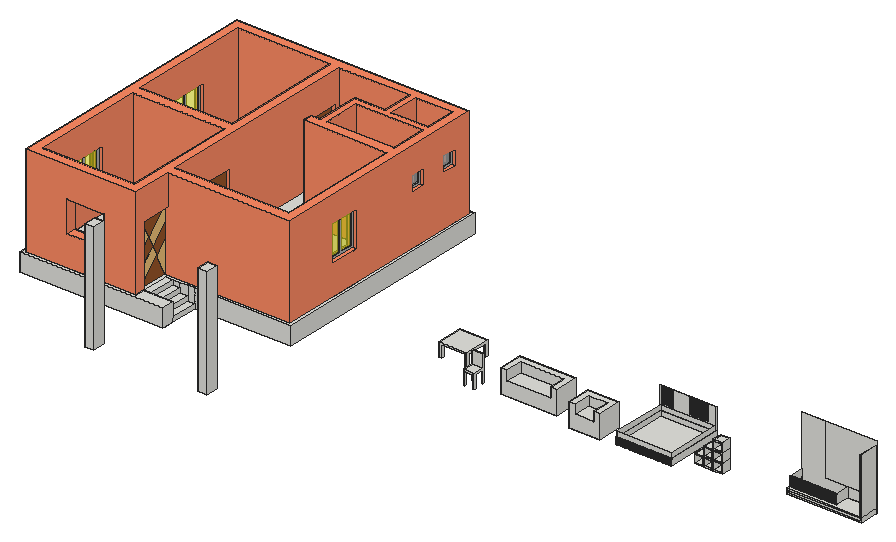
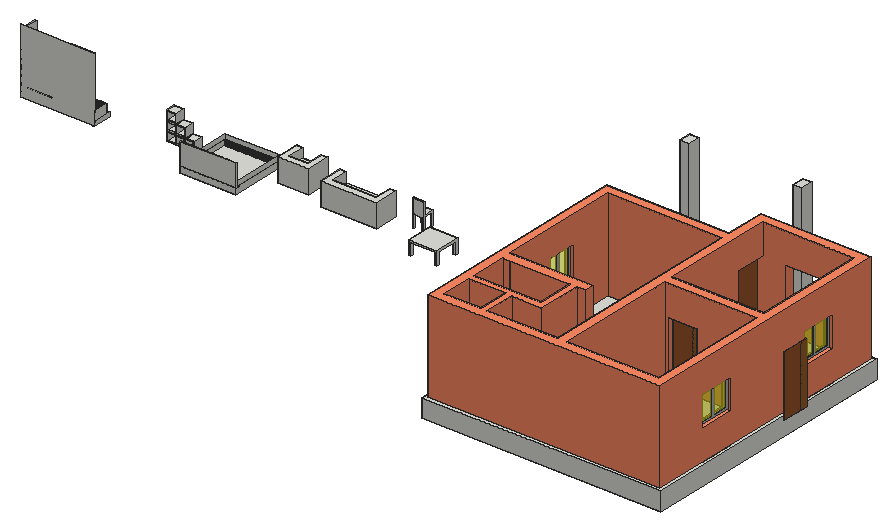
# SketchUp Ruby script. Lengths in inches.
U = 1.inch
M = Sketchup.active_model
def pt(a) = Geom::Point3d.new(a.map { |v| v * U })
def face(e, loops, mat)
  f = e.add_face(loops[0].map { |a| pt(a) })
  loops[1..].each { |l| e.add_face(l.map { |a| pt(a) }).erase! }
  f.material = f.back_material = mat if mat
  f
end
# faces: each face lists its corners as indices into pts; further lists are holes
def faces(e, pts, list, mat = nil) = list.each { |f| face(e, (f[0].is_a?(Array) ? f : [f]).map { |l| l.map { |i| pts[i] } }, mat) }
# xy, xz, yz: faces in a plane at the given z, y or x. An outline is a flat list of corners, or four numbers for a rectangle; further outlines are holes
def ring(l) = l.size == 4 ? [[l[0], l[1]], [l[2], l[1]], [l[2], l[3]], [l[0], l[3]]] : l.each_slice(2).to_a
def flat(e, list, mat, &to3) = list.each { |f| face(e, (f[0].is_a?(Array) ? f : [f]).map { |l| ring(l).map { |u, v| to3.(u, v) } }, mat) }
def xy(e, z, list, mat = nil) = flat(e, list, mat) { |x, y| [x, y, z] }
def xz(e, y, list, mat = nil) = flat(e, list, mat) { |x, z| [x, y, z] }
def yz(e, x, list, mat = nil) = flat(e, list, mat) { |y, z| [x, y, z] }
def lines(e, pts, list) = list.each { |a, b| e.add_line(pt(pts[a]), pt(pts[b])) }
# prism: a flat outline (further loops are holes) pulled along v
def prism(e, loops, v, mat = nil)
  f = face(e, loops, mat); d = Geom::Vector3d.new(v.map { |x| x * U })
  f.pushpull(f.normal.samedirection?(d) ? d.length : -d.length)
end
def box(e, o, s, mat = nil) = prism(e, [[o, [o[0] + s[0], o[1], o[2]], [o[0] + s[0], o[1] + s[1], o[2]], [o[0], o[1] + s[1], o[2]]]], [0, 0, s[2]], mat)
def at(x, y, z, deg = 0) = Geom::Transformation.translation(pt([x, y, z])) * Geom::Transformation.rotation(ORIGIN, Z_AXIS, deg.degrees)
def axes(o, x, y, z) = Geom::Transformation.new([*x, 0, *y, 0, *z, 0, *pt(o).to_a, 1])
def part(name) = M.definitions.add(name)
# library, detail: a bought-in or finely detailed component or shape, given as its bounding box
def library(name, o, s) = part(name).tap { |d| box(d.entities, o, s) }
def detail(e, o, s) = box(e.add_group.entities, o, s)
def put(e, d, t, mat = nil) = e.add_instance(d, t).tap { |i| i.material = mat if mat }
def group(e, t, mat = nil) = e.add_group.tap { |g| g.transformation = t; g.material = mat if mat }.entities
root = M.entities
M.materials.add("[Aluminum]").color = [179, 179, 179]
M.materials.add("[Color B03]").color = [255, 140, 101]
M.materials.add("[Translucent Glass Gold]").color = [255, 254, 26]
M.materials["[Translucent Glass Gold]"].alpha = 0.6
M.materials.add("[Translucent Resin Crush Gray]").color = [184, 184, 184]
M.materials["[Translucent Resin Crush Gray]"].alpha = 0.8
M.materials.add("[Wood Cherry Original]").color = [152, 86, 42]
M.materials.add("[Wood Floor Dark]").color = [153, 94, 42]
M.materials.add("[Wood Floor]").color = [155, 105, 61]
M.materials.add("[Wood OSB]").color = [240, 195, 122]
c1 = part("Group\#23")
box(c1.entities,[0,0,-141.73],[11.8125,15.75,141.73])
c2 = part("Group\#17")
xy(c2.entities,0,[[0,0,0.98,35.43]],"[Wood Cherry Original]")
xy(c2.entities,78.74,[[0,8.88,0.98,35.43]],"[Wood Cherry Original]")
xy(c2.entities,78.74,[[0,0,0.98,8.88]],"[Wood Floor Dark]")
xz(c2.entities,0,[[0,0,0.98,78.74]],"[Wood Cherry Original]")
xz(c2.entities,35.43,[[0,0,0.98,78.74]],"[Wood Cherry Original]")
yz(c2.entities,0,[[8.88,0,35.43,78.74]],"[Wood Cherry Original]")
yz(c2.entities,0,[[0,0,8.88,78.74]],"[Wood Floor Dark]")
yz(c2.entities,0.98,[[8.88,0,35.43,78.74]],"[Wood Cherry Original]")
yz(c2.entities,0.98,[[0,0,8.88,78.74]],"[Wood Floor Dark]")
c3 = part("Group\#14")
prism(c3.entities,[[[0,47.24,39.37],[0,47.24,0],[0,0,0],[0,0,39.37]],[[0,1.97,1.97],[0,22.64,1.97],[0,22.64,37.4],[0,1.97,37.4]],[[0,24.61,37.4],[0,24.61,1.97],[0,45.28,1.97],[0,45.28,37.4]]],[1.97,0,0])
c4 = part("Group\#4")
p = [[0,3.9375,0],[47.24,3.9375,0],[0,7.875,0],[47.24,7.875,0],[47.24,11.8125,0],[47.24,0,0],
  [0,11.8125,0],[0,0,0]]
lines(c4.entities,p,[[0,1],[2,0],[3,4],[5,1],[4,6],[2,3],[6,2],[1,3],[7,5],[0,7]])
c5 = part("Group\#8")
xy(c5.entities,0,[[0,0,11.8125,19.69]])
p = [[3.9375,19.69,0],[3.9375,17.9,0],[3.9375,16.11,0],[3.9375,14.32,0],[3.9375,12.53,0],[3.9375,10.74,0],
  [3.9375,8.95,0],[3.9375,7.16,0],[3.9375,5.37,0],[3.9375,3.58,0],[3.9375,1.79,0],[3.9375,0,0],
  [7.875,5.37,0],[7.875,3.58,0],[7.875,8.95,0],[7.875,7.16,0],[7.875,16.11,0],[7.875,14.32,0],
  [7.875,12.53,0],[7.875,10.74,0],[7.875,1.79,0],[7.875,0,0],[7.875,19.69,0],[7.875,17.9,0]]
lines(c5.entities,p,[[0,1],[2,3],[4,5],[6,7],[8,9],[10,11],[12,13],[14,15],[16,17],[18,19],[20,21],[22,23]])
c6 = part("Group\#16")
yz(c6.entities,0.98,[[1.97,1.97,17.72,17.72]],"[Translucent Resin Crush Gray]")
g1 = group(c6.entities,at(0,0,0),"[Aluminum]")
prism(g1,[[[1.97,19.69,0],[1.97,19.69,19.69],[1.97,0,19.69],[1.97,0,0]],[[1.97,1.97,17.72],[1.97,17.72,17.72],[1.97,17.72,1.97],[1.97,1.97,1.97]]],[-1.97,0,0])
c7 = part("Group\#7")
p = [[11.8125,0,0],[11.8125,19.69,0],[0,19.69,0],[0,0,0]]
lines(c7.entities,p,[[0,1],[1,2],[2,3],[3,0]])
g2 = group(c7.entities,at(0,0,0))
p = [[0,0,0],[11.8125,0,0],[11.8125,19.69,0],[0,19.69,0]]
lines(g2,p,[[0,1],[2,3],[3,0],[1,2]])
c8 = part("Group\#19")
xy(c8.entities,0,[[0,0,1.97,31.5]])
xy(c8.entities,1.97,[[0,1.97,1.97,29.53]])
xy(c8.entities,76.77,[[0,1.97,1.97,29.53]])
xy(c8.entities,78.74,[[0,0,1.97,31.5]],"[Wood OSB]")
xz(c8.entities,0,[[0,0,1.97,78.74]])
xz(c8.entities,1.97,[[0,1.97,1.97,76.77]])
xz(c8.entities,29.53,[[0,1.97,1.97,76.77]])
xz(c8.entities,31.5,[[0,0,1.97,78.74]])
yz(c8.entities,0,[[[0,0,31.5,78.74],[1.97,1.97,29.53,76.77]]],"[Wood OSB]")
yz(c8.entities,1.97,[[1.97,1.97,29.53,76.77]],"[Wood Floor]")
yz(c8.entities,1.97,[[[0,0,31.5,78.74],[1.97,1.97,29.53,76.77]]],"[Wood OSB]")
c9 = part("Component\#7")
xy(c9.entities,0,[[0,0,40,30]])
xy(c9.entities,18,[[8,0,32,22]])
xy(c9.entities,30,[[0,0,8,0,8,22,32,22,32,0,40,0,40,30,0,30]])
xz(c9.entities,0,[[0,0,40,0,40,30,32,30,32,18,8,18,8,30,0,30]])
xz(c9.entities,22,[[8,18,32,30]])
xz(c9.entities,30,[[0,0,40,30]])
yz(c9.entities,0,[[0,0,30,30]])
yz(c9.entities,8,[[0,18,22,30]])
yz(c9.entities,32,[[0,18,22,30]])
yz(c9.entities,40,[[0,0,30,30]])
xy(root,0,[[524.43,143.5,526.43,145.5],[536.43,143.5,538.43,145.5],[718.98,144.73,720.98,145.23],[721.48,144.73,723.48,145.23],[723.98,144.73,725.98,145.23],
  [726.48,144.73,728.48,145.23],[728.98,144.73,730.98,145.23],[731.48,144.73,733.48,145.23],[733.98,144.73,735.98,145.23],[736.48,144.73,738.48,145.23],
  [738.98,144.73,740.98,145.23],[741.48,144.73,743.48,145.23],[743.98,144.73,745.98,145.23],[746.48,144.73,748.48,145.23],[748.98,144.73,750.98,145.23],
  [751.48,144.73,753.48,145.23],[753.98,144.73,755.98,145.23],[756.48,144.73,758.48,145.23],[758.98,144.73,760.98,145.23],[761.48,144.73,763.48,145.23],
  [763.98,144.73,765.98,145.23],[766.48,144.73,768.48,145.23],[768.98,144.73,770.98,145.23],[771.48,144.73,773.48,145.23],[773.98,144.73,775.98,145.23],
  [776.48,144.73,778.48,145.23],[778.98,144.73,780.98,145.23],[781.48,144.73,783.48,145.23],[783.98,144.73,785.98,145.23],[786.48,144.73,788.48,145.23],
  [788.98,144.73,790.98,145.23],[718.98,145.23,790.98,217.23],[564.9,153.125,636.9,183.125],[524.43,157.5,526.43,159.5],[536.43,157.5,538.43,159.5],
  [805.82,163.28,817.82,175.28],[817.82,163.28,829.82,175.28],[829.82,163.28,841.82,175.28],[917.17,172.59,1013.17,196.09],[470.13,172.67,473.13,175.67],
  [503.13,172.67,506.13,175.67],[917.17,196.09,1013.17,196.59],[470.13,202.67,473.13,205.67],[503.13,202.67,506.13,205.67]])
xy(root,1,[[806.82,163.28,816.82,175.28],[818.82,163.28,828.82,175.28],[830.82,163.28,840.82,175.28]])
xy(root,6,[[[917.17,172.59,1011.17,172.59,1013.17,196.09,917.17,196.09,917.17,178.59,919.17,178.59,919.17,178.09,917.17,178.09],[919.67,178.09,921.67,178.59],[922.17,178.09,924.17,178.59],[924.67,178.09,926.67,178.59],[927.17,178.09,929.17,178.59],[929.67,178.09,931.67,178.59],[932.17,178.09,934.17,178.59],[934.67,178.09,936.67,178.59],[937.17,178.09,939.17,178.59],[939.67,178.09,941.67,178.59],[942.17,178.09,944.17,178.59],[944.67,178.09,946.67,178.59],[947.17,178.09,949.17,178.59],[949.67,178.09,951.67,178.59],[952.17,178.09,954.17,178.59],[954.67,178.09,956.67,178.59],[957.17,178.09,959.17,178.59],[959.67,178.09,961.67,178.59],[962.17,178.09,964.17,178.59],[964.67,178.09,966.67,178.59],[967.17,178.09,969.17,178.59],[969.67,178.09,971.67,178.59],[972.17,178.09,974.17,178.59],[974.67,178.09,976.67,178.59]],[1011.17,172.59,1013.17,172.59,1013.17,196.09],[917.17,178.09,919.17,178.59],[919.67,178.09,921.67,178.59],[922.17,178.09,924.17,178.59],
  [924.67,178.09,926.67,178.59],[927.17,178.09,929.17,178.59],[929.67,178.09,931.67,178.59],[932.17,178.09,934.17,178.59],[934.67,178.09,936.67,178.59],
  [937.17,178.09,939.17,178.59],[939.67,178.09,941.67,178.59],[942.17,178.09,944.17,178.59],[944.67,178.09,946.67,178.59],[947.17,178.09,949.17,178.59],
  [949.67,178.09,951.67,178.59],[952.17,178.09,954.17,178.59],[954.67,178.09,956.67,178.59],[957.17,178.09,959.17,178.59],[959.67,178.09,961.67,178.59],
  [962.17,178.09,964.17,178.59],[964.67,178.09,966.67,178.59],[967.17,178.09,969.17,178.59],[969.67,178.09,971.67,178.59],[972.17,178.09,974.17,178.59],
  [974.67,178.09,976.67,178.59]])
xy(root,8,[[718.98,144.73,720.98,145.23],[721.48,144.73,723.48,145.23],[723.98,144.73,725.98,145.23],[726.48,144.73,728.48,145.23],[728.98,144.73,730.98,145.23],
  [731.48,144.73,733.48,145.23],[733.98,144.73,735.98,145.23],[736.48,144.73,738.48,145.23],[738.98,144.73,740.98,145.23],[741.48,144.73,743.48,145.23],
  [743.98,144.73,745.98,145.23],[746.48,144.73,748.48,145.23],[748.98,144.73,750.98,145.23],[751.48,144.73,753.48,145.23],[753.98,144.73,755.98,145.23],
  [756.48,144.73,758.48,145.23],[758.98,144.73,760.98,145.23],[761.48,144.73,763.48,145.23],[763.98,144.73,765.98,145.23],[766.48,144.73,768.48,145.23],
  [768.98,144.73,770.98,145.23],[771.48,144.73,773.48,145.23],[773.98,144.73,775.98,145.23],[776.48,144.73,778.48,145.23],[778.98,144.73,780.98,145.23],
  [781.48,144.73,783.48,145.23],[783.98,144.73,785.98,145.23],[786.48,144.73,788.48,145.23],[788.98,144.73,790.98,145.23],[[718.98,145.23,790.98,216.73],[719.98,146.23,789.98,216.23]],
  [718.98,216.73,790.98,217.23]])
xy(root,11,[[806.82,163.28,816.82,175.28],[818.82,163.28,828.82,175.28],[830.82,163.28,840.82,175.28]])
xy(root,12,[[805.82,163.28,817.82,175.28],[817.82,163.28,829.82,175.28],[829.82,163.28,841.82,175.28]])
xy(root,13,[[818.82,163.28,828.82,175.28],[830.82,163.28,840.82,175.28]])
xy(root,15,[[473.13,172.67,473.13,175.67,470.13,175.67,470.13,202.67,473.13,202.67,473.13,205.67,503.13,205.67,503.13,202.67,506.13,202.67,506.13,175.67,503.13,175.67,503.13,172.67]])
xy(root,16,[[526.43,143.5,526.43,145.5,524.43,145.5,524.43,157.5,526.43,157.5,526.43,159.5,536.43,159.5,536.43,157.5,538.43,157.5,538.43,145.5,536.43,145.5,536.43,143.5]])
xy(root,17.5,[[572.9,153.125,628.9,175.125]])
xy(root,18,[[524.43,143.5,538.43,157.5],[470.13,172.67,506.13,205.67]])
xy(root,23,[[818.82,163.28,828.82,175.28],[830.82,163.28,840.82,175.28]])
xy(root,24,[[817.82,163.28,829.82,175.28],[829.82,163.28,841.82,175.28]])
xy(root,25,[[830.82,163.28,840.82,175.28]])
xy(root,30,[[564.9,153.125,572.9,153.125,572.9,175.125,628.9,175.125,628.9,153.125,636.9,153.125,636.9,183.125,564.9,183.125]])
xy(root,34,[[524.43,157.5,538.43,159.5]])
xy(root,35,[[830.82,163.28,840.82,175.28]])
xy(root,36,[[829.82,163.28,841.82,175.28]])
xz(root,143.5,[[524.43,0,526.43,0,526.43,16,536.43,16,536.43,0,538.43,0,538.43,18,524.43,18]])
xz(root,144.73,[[718.98,0,720.98,8],[721.48,0,723.48,8],[723.98,0,725.98,8],[726.48,0,728.48,8],[728.98,0,730.98,8],
  [731.48,0,733.48,8],[733.98,0,735.98,8],[736.48,0,738.48,8],[738.98,0,740.98,8],[741.48,0,743.48,8],
  [743.98,0,745.98,8],[746.48,0,748.48,8],[748.98,0,750.98,8],[751.48,0,753.48,8],[753.98,0,755.98,8],
  [756.48,0,758.48,8],[758.98,0,760.98,8],[761.48,0,763.48,8],[763.98,0,765.98,8],[766.48,0,768.48,8],
  [768.98,0,770.98,8],[771.48,0,773.48,8],[773.98,0,775.98,8],[776.48,0,778.48,8],[778.98,0,780.98,8],
  [781.48,0,783.48,8],[783.98,0,785.98,8],[786.48,0,788.48,8],[788.98,0,790.98,8]])
xz(root,145.23,[[718.98,0,720.98,8],[720.98,0,721.48,8],[721.48,0,723.48,8],[723.48,0,723.98,8],[723.98,0,725.98,8],
  [725.98,0,726.48,8],[726.48,0,728.48,8],[728.48,0,728.98,8],[728.98,0,730.98,8],[730.98,0,731.48,8],
  [731.48,0,733.48,8],[733.48,0,733.98,8],[733.98,0,735.98,8],[735.98,0,736.48,8],[736.48,0,738.48,8],
  [738.48,0,738.98,8],[738.98,0,740.98,8],[740.98,0,741.48,8],[741.48,0,743.48,8],[743.48,0,743.98,8],
  [743.98,0,745.98,8],[745.98,0,746.48,8],[746.48,0,748.48,8],[748.48,0,748.98,8],[748.98,0,750.98,8],
  [750.98,0,751.48,8],[751.48,0,753.48,8],[753.48,0,753.98,8],[753.98,0,755.98,8],[755.98,0,756.48,8],
  [756.48,0,758.48,8],[758.48,0,758.98,8],[758.98,0,760.98,8],[760.98,0,761.48,8],[761.48,0,763.48,8],
  [763.48,0,763.98,8],[763.98,0,765.98,8],[765.98,0,766.48,8],[766.48,0,768.48,8],[768.48,0,768.98,8],
  [768.98,0,770.98,8],[770.98,0,771.48,8],[771.48,0,773.48,8],[773.48,0,773.98,8],[773.98,0,775.98,8],
  [775.98,0,776.48,8],[776.48,0,778.48,8],[778.48,0,778.98,8],[778.98,0,780.98,8],[780.98,0,781.48,8],
  [781.48,0,783.48,8],[783.48,0,783.98,8],[783.98,0,785.98,8],[785.98,0,786.48,8],[786.48,0,788.48,8],
  [788.48,0,788.98,8],[788.98,0,790.98,8]])
xz(root,145.5,[[524.43,0,526.43,16],[536.43,0,538.43,16]])
xz(root,146.23,[[719.98,8,789.98,14]])
xz(root,153.125,[[564.9,0,636.9,0,636.9,30,628.9,30,628.9,17.5,572.9,17.5,572.9,30,564.9,30]])
xz(root,157.5,[[524.43,0,526.43,16],[536.43,0,538.43,16],[524.43,18,538.43,34]])
xz(root,159.5,[[524.43,0,524.43,34,538.43,34,538.43,0,536.43,0,536.43,16,526.43,16,526.43,0]])
xz(root,163.28,[[[805.82,0,817.82,12],[806.82,1,816.82,11]],[[817.82,0,829.82,12],[818.82,1,828.82,11]],[[829.82,0,841.82,12],[830.82,1,840.82,11]],[[817.82,12,829.82,24],[818.82,13,828.82,23]],[[829.82,12,841.82,24],[830.82,13,840.82,23]],
  [[829.82,24,841.82,36],[830.82,25,840.82,35]]])
xz(root,172.59,[[[917.17,0,1013.17,6],[918.17,1,1012.17,5]],[918.17,1,1012.17,5],[[1011.17,6,1013.17,78],[1011.67,6.5,1012.67,77.5]],[1011.67,6.5,1012.67,77.5]])
xz(root,172.67,[[470.13,0,473.13,0,473.13,15,503.13,15,503.13,0,506.13,0,506.13,18,470.13,18]])
xz(root,175.125,[[572.9,17.5,628.9,30]])
xz(root,175.28,[[[805.82,0,817.82,12],[806.82,1,816.82,11]],[[817.82,0,829.82,12],[818.82,1,828.82,11]],[[829.82,0,841.82,12],[830.82,1,840.82,11]],[[817.82,12,829.82,24],[818.82,13,828.82,23]],[[829.82,12,841.82,24],[830.82,13,840.82,23]],
  [[829.82,24,841.82,36],[830.82,25,840.82,35]]])
xz(root,175.67,[[470.13,0,473.13,15],[503.13,0,506.13,15]])
xz(root,178.09,[[917.17,6,919.17,18],[919.67,6,921.67,18],[922.17,6,924.17,18],[924.67,6,926.67,18],[927.17,6,929.17,18],
  [929.67,6,931.67,18],[932.17,6,934.17,18],[934.67,6,936.67,18],[937.17,6,939.17,18],[939.67,6,941.67,18],
  [942.17,6,944.17,18],[944.67,6,946.67,18],[947.17,6,949.17,18],[949.67,6,951.67,18],[952.17,6,954.17,18],
  [954.67,6,956.67,18],[957.17,6,959.17,18],[959.67,6,961.67,18],[962.17,6,964.17,18],[964.67,6,966.67,18],
  [967.17,6,969.17,18],[969.67,6,971.67,18],[972.17,6,974.17,18],[974.67,6,976.67,18]])
xz(root,178.59,[[917.17,6,919.17,18],[919.17,6,919.67,18],[919.67,6,921.67,18],[921.67,6,922.17,18],[922.17,6,924.17,18],
  [924.17,6,924.67,18],[924.67,6,926.67,18],[926.67,6,927.17,18],[927.17,6,929.17,18],[929.17,6,929.67,18],
  [929.67,6,931.67,18],[931.67,6,932.17,18],[932.17,6,934.17,18],[934.17,6,934.67,18],[934.67,6,936.67,18],
  [936.67,6,937.17,18],[937.17,6,939.17,18],[939.17,6,939.67,18],[939.67,6,941.67,18],[941.67,6,942.17,18],
  [942.17,6,944.17,18],[944.17,6,944.67,18],[944.67,6,946.67,18],[946.67,6,947.17,18],[947.17,6,949.17,18],
  [949.17,6,949.67,18],[949.67,6,951.67,18],[951.67,6,952.17,18],[952.17,6,954.17,18],[954.17,6,954.67,18],
  [954.67,6,956.67,18],[956.67,6,957.17,18],[957.17,6,959.17,18],[959.17,6,959.67,18],[959.67,6,961.67,18],
  [961.67,6,962.17,18],[962.17,6,964.17,18],[964.17,6,964.67,18],[964.67,6,966.67,18],[966.67,6,967.17,18],
  [967.17,6,969.17,18],[969.17,6,969.67,18],[969.67,6,971.67,18],[971.67,6,972.17,18],[972.17,6,974.17,18],
  [974.17,6,974.67,18],[974.67,6,976.67,18],[976.67,6,977.17,18]])
xz(root,183.125,[[564.9,0,636.9,30]])
xz(root,196.09,[[917.17,0,1013.17,6],[917.17,6,977.17,6,977.17,18,947.17,18,947.17,84,917.17,84],[977.17,6,1013.17,18]])
xz(root,196.59,[[[917.17,0,1013.17,84],[971.17,13.08,1011.17,15.08]]])
xz(root,202.67,[[470.13,0,473.13,15],[503.13,0,506.13,15]])
xz(root,205.67,[[470.13,0,470.13,18,506.13,18,506.13,0,503.13,0,503.13,15,473.13,15,473.13,0]])
xz(root,216.23,[[719.98,8,789.98,14]])
xz(root,216.73,[[718.98,8,790.98,8,790.98,14,788.98,14,788.98,36,788.48,36,788.48,14,786.48,14,786.48,36,785.98,36,785.98,14,783.98,14,783.98,36,783.48,36,783.48,14,781.48,14,781.48,36,780.98,36,780.98,14,778.98,14,778.98,36,778.48,36,778.48,14,776.48,14,776.48,36,775.98,36,775.98,14,773.98,14,773.98,36,773.48,36,773.48,14,771.48,14,771.48,36,770.98,36,770.98,14,768.98,14,768.98,36,768.48,36,768.48,14,766.48,14,766.48,36,765.98,36,765.98,14,763.98,14,763.98,36,763.48,36,763.48,14,761.48,14,761.48,36,760.98,36,760.98,14,758.98,14,758.98,36,758.48,36,758.48,14,756.48,14,756.48,36,755.98,36,755.98,14,753.98,14,753.98,36,753.48,36,753.48,14,751.48,14,751.48,36,750.98,36,750.98,14,748.98,14,748.98,36,748.48,36,748.48,14,746.48,14,746.48,36,745.98,36,745.98,14,743.98,14,743.98,36,743.48,36,743.48,14,741.48,14,741.48,36,740.98,36,740.98,14,738.98,14,738.98,36,738.48,36,738.48,14,736.48,14,736.48,36,735.98,36,735.98,14,733.98,14,733.98,36,733.48,36,733.48,14,731.48,14,731.48,36,730.98,36,730.98,14,728.98,14,728.98,36,728.48,36,728.48,14,726.48,14,726.48,36,725.98,36,725.98,14,723.98,14,723.98,36,723.48,36,723.48,14,721.48,14,721.48,36,720.98,36,720.98,14,718.98,14]])
xz(root,217.23,[[718.98,0,790.98,8],[718.98,8,790.98,36]])
yz(root,470.13,[[172.67,0,172.67,18,205.67,18,205.67,0,202.67,0,202.67,15,175.67,15,175.67,0]])
yz(root,473.13,[[172.67,0,175.67,15],[202.67,0,205.67,15]])
yz(root,503.13,[[172.67,0,175.67,15],[202.67,0,205.67,15]])
yz(root,506.13,[[172.67,0,175.67,0,175.67,15,202.67,15,202.67,0,205.67,0,205.67,18,172.67,18]])
yz(root,524.43,[[143.5,0,143.5,18,157.5,18,157.5,34,159.5,34,159.5,0,157.5,0,157.5,16,145.5,16,145.5,0]])
yz(root,526.43,[[143.5,0,145.5,16],[157.5,0,159.5,16]])
yz(root,536.43,[[143.5,0,145.5,16],[157.5,0,159.5,16]])
yz(root,538.43,[[143.5,0,145.5,0,145.5,16,157.5,16,157.5,0,159.5,0,159.5,34,157.5,34,157.5,18,143.5,18]])
yz(root,564.9,[[153.125,0,183.125,30]])
yz(root,572.9,[[153.125,17.5,175.125,30]])
yz(root,628.9,[[153.125,17.5,175.125,30]])
yz(root,636.9,[[153.125,0,183.125,30]])
yz(root,718.98,[[144.73,0,145.23,8],[145.23,0,217.23,8],[216.73,8,217.23,36]])
yz(root,719.98,[[146.23,8,216.23,14]])
yz(root,720.98,[[144.73,0,145.23,8]])
yz(root,721.48,[[144.73,0,145.23,8]])
yz(root,723.48,[[144.73,0,145.23,8]])
yz(root,723.98,[[144.73,0,145.23,8]])
yz(root,725.98,[[144.73,0,145.23,8]])
yz(root,726.48,[[144.73,0,145.23,8]])
yz(root,728.48,[[144.73,0,145.23,8]])
yz(root,728.98,[[144.73,0,145.23,8]])
yz(root,730.98,[[144.73,0,145.23,8]])
yz(root,731.48,[[144.73,0,145.23,8]])
yz(root,733.48,[[144.73,0,145.23,8]])
yz(root,733.98,[[144.73,0,145.23,8]])
yz(root,735.98,[[144.73,0,145.23,8]])
yz(root,736.48,[[144.73,0,145.23,8]])
yz(root,738.48,[[144.73,0,145.23,8]])
yz(root,738.98,[[144.73,0,145.23,8]])
yz(root,740.98,[[144.73,0,145.23,8]])
yz(root,741.48,[[144.73,0,145.23,8]])
yz(root,743.48,[[144.73,0,145.23,8]])
yz(root,743.98,[[144.73,0,145.23,8]])
yz(root,745.98,[[144.73,0,145.23,8]])
yz(root,746.48,[[144.73,0,145.23,8]])
yz(root,748.48,[[144.73,0,145.23,8]])
yz(root,748.98,[[144.73,0,145.23,8]])
yz(root,750.98,[[144.73,0,145.23,8]])
yz(root,751.48,[[144.73,0,145.23,8]])
yz(root,753.48,[[144.73,0,145.23,8]])
yz(root,753.98,[[144.73,0,145.23,8]])
yz(root,755.98,[[144.73,0,145.23,8]])
yz(root,756.48,[[144.73,0,145.23,8]])
yz(root,758.48,[[144.73,0,145.23,8]])
yz(root,758.98,[[144.73,0,145.23,8]])
yz(root,760.98,[[144.73,0,145.23,8]])
yz(root,761.48,[[144.73,0,145.23,8]])
yz(root,763.48,[[144.73,0,145.23,8]])
yz(root,763.98,[[144.73,0,145.23,8]])
yz(root,765.98,[[144.73,0,145.23,8]])
yz(root,766.48,[[144.73,0,145.23,8]])
yz(root,768.48,[[144.73,0,145.23,8]])
yz(root,768.98,[[144.73,0,145.23,8]])
yz(root,770.98,[[144.73,0,145.23,8]])
yz(root,771.48,[[144.73,0,145.23,8]])
yz(root,773.48,[[144.73,0,145.23,8]])
yz(root,773.98,[[144.73,0,145.23,8]])
yz(root,775.98,[[144.73,0,145.23,8]])
yz(root,776.48,[[144.73,0,145.23,8]])
yz(root,778.48,[[144.73,0,145.23,8]])
yz(root,778.98,[[144.73,0,145.23,8]])
yz(root,780.98,[[144.73,0,145.23,8]])
yz(root,781.48,[[144.73,0,145.23,8]])
yz(root,783.48,[[144.73,0,145.23,8]])
yz(root,783.98,[[144.73,0,145.23,8]])
yz(root,785.98,[[144.73,0,145.23,8]])
yz(root,786.48,[[144.73,0,145.23,8]])
yz(root,788.48,[[144.73,0,145.23,8]])
yz(root,788.98,[[144.73,0,145.23,8]])
yz(root,789.98,[[146.23,8,216.23,14]])
yz(root,790.98,[[144.73,0,145.23,8],[145.23,0,217.23,8],[216.73,8,217.23,36]])
yz(root,805.82,[[163.28,0,175.28,12]])
yz(root,806.82,[[163.28,1,175.28,11]])
yz(root,816.82,[[163.28,1,175.28,11]])
yz(root,817.82,[[163.28,0,175.28,12],[163.28,12,175.28,24]])
yz(root,818.82,[[163.28,1,175.28,11],[163.28,13,175.28,23]])
yz(root,828.82,[[163.28,1,175.28,11],[163.28,13,175.28,23]])
yz(root,829.82,[[163.28,0,175.28,12],[163.28,12,175.28,24],[163.28,24,175.28,36]])
yz(root,830.82,[[163.28,1,175.28,11],[163.28,13,175.28,23],[163.28,25,175.28,35]])
yz(root,840.82,[[163.28,1,175.28,11],[163.28,13,175.28,23],[163.28,25,175.28,35]])
yz(root,841.82,[[163.28,0,175.28,12],[163.28,12,175.28,24],[163.28,24,175.28,36]])
yz(root,917.17,[[172.59,0,196.09,6],[196.09,0,196.59,6],[178.09,6,178.59,18],[178.59,6,196.09,18],[196.09,6,196.59,18]])
yz(root,919.17,[[178.09,6,178.59,18]])
yz(root,919.67,[[178.09,6,178.59,18]])
yz(root,921.67,[[178.09,6,178.59,18]])
yz(root,922.17,[[178.09,6,178.59,18]])
yz(root,924.17,[[178.09,6,178.59,18]])
yz(root,924.67,[[178.09,6,178.59,18]])
yz(root,926.67,[[178.09,6,178.59,18]])
yz(root,927.17,[[178.09,6,178.59,18]])
yz(root,929.17,[[178.09,6,178.59,18]])
yz(root,929.67,[[178.09,6,178.59,18]])
yz(root,931.67,[[178.09,6,178.59,18]])
yz(root,932.17,[[178.09,6,178.59,18]])
yz(root,934.17,[[178.09,6,178.59,18]])
yz(root,934.67,[[178.09,6,178.59,18]])
yz(root,936.67,[[178.09,6,178.59,18]])
yz(root,937.17,[[178.09,6,178.59,18]])
yz(root,939.17,[[178.09,6,178.59,18]])
yz(root,939.67,[[178.09,6,178.59,18]])
yz(root,941.67,[[178.09,6,178.59,18]])
yz(root,942.17,[[178.09,6,178.59,18]])
yz(root,944.17,[[178.09,6,178.59,18]])
yz(root,944.67,[[178.09,6,178.59,18]])
yz(root,946.67,[[178.09,6,178.59,18]])
yz(root,947.17,[[178.09,6,178.59,18]])
yz(root,949.17,[[178.09,6,178.59,18]])
yz(root,949.67,[[178.09,6,178.59,18]])
yz(root,951.67,[[178.09,6,178.59,18]])
yz(root,952.17,[[178.09,6,178.59,18]])
yz(root,954.17,[[178.09,6,178.59,18]])
yz(root,954.67,[[178.09,6,178.59,18]])
yz(root,956.67,[[178.09,6,178.59,18]])
yz(root,957.17,[[178.09,6,178.59,18]])
yz(root,959.17,[[178.09,6,178.59,18]])
yz(root,959.67,[[178.09,6,178.59,18]])
yz(root,961.67,[[178.09,6,178.59,18]])
yz(root,962.17,[[178.09,6,178.59,18]])
yz(root,964.17,[[178.09,6,178.59,18]])
yz(root,964.67,[[178.09,6,178.59,18]])
yz(root,966.67,[[178.09,6,178.59,18]])
yz(root,967.17,[[178.09,6,178.59,18]])
yz(root,969.17,[[178.09,6,178.59,18]])
yz(root,969.67,[[178.09,6,178.59,18]])
yz(root,971.67,[[178.09,6,178.59,18]])
yz(root,972.17,[[178.09,6,178.59,18]])
yz(root,974.17,[[178.09,6,178.59,18]])
yz(root,974.67,[[178.09,6,178.59,18]])
yz(root,976.67,[[178.09,6,178.59,18]])
yz(root,977.17,[[178.59,6,196.09,18]])
yz(root,1013.17,[[172.59,0,196.09,6],[196.09,0,196.59,6],[172.59,6,196.09,78],[196.09,6,196.59,78]])
p = [[1013.17,196.09,6],[1011.17,172.59,6],[1011.17,172.59,13.08],[1011.17,172.59,15.08],[1011.17,172.59,78],[1013.17,196.09,78],
  [1013.17,196.09,18]]
faces(root,p,[[0,1,2,3,4,5,6]])
g3 = group(root,at(6.4,78.74,0))
xy(g3,-23.62,[[0,0,0,346.46,307.09,346.46,307.09,51.18,183.46,51.18,183.46,15.75,145.67,15.75,145.67,3.9375,183.46,3.9375,183.46,0],[145.67,3.9375,183.46,15.75]])
xy(g3,-17.72,[[174.02,15.75,183.46,51.18]])
xy(g3,-11.8125,[[164.57,15.75,174.02,51.18]])
xy(g3,-5.91,[[155.12,15.75,164.57,51.18]])
xy(g3,0,[[0,0,183.46,0,183.46,15.75,145.67,15.75,145.67,51.18,307.09,51.18,307.09,346.46,0,346.46],[145.67,15.75,155.12,51.18]])
xz(g3,0,[[0,-23.62,183.46,0]])
xz(g3,15.75,[[145.67,-23.62,155.12,0],[155.12,-23.62,164.57,-5.91],[164.57,-23.62,174.02,-11.8125],[174.02,-23.62,183.46,-17.72],[174.02,-17.72,174.02,-11.8125,164.57,-11.8125,164.57,-5.91,155.12,-5.91,155.12,0,183.46,0,183.46,-17.72]])
xz(g3,51.18,[[183.46,-23.62,307.09,0],[174.02,-17.72,183.46,0],[164.57,-11.8125,174.02,0],[155.12,-5.91,164.57,0]])
xz(g3,346.46,[[0,-23.62,307.09,0]])
yz(g3,0,[[0,-23.62,346.46,0]])
yz(g3,145.67,[[3.9375,-23.62,15.75,0]])
yz(g3,155.12,[[15.75,-5.91,51.18,0]])
yz(g3,164.57,[[15.75,-11.8125,51.18,-5.91]])
yz(g3,174.02,[[15.75,-17.72,51.18,-11.8125]])
yz(g3,183.46,[[0,-23.62,15.75,0],[15.75,-23.62,51.18,-17.72]])
yz(g3,307.09,[[51.18,-23.62,346.46,0]])
put(root,c1,at(297.74,0,118.11))
put(root,c1,at(152.07,0,118.11))
g4 = group(root,at(147.15,94.49,0))
xy(g4,0,[[0,0,0.98,39.37]],"[Wood Cherry Original]")
xy(g4,78.74,[[0,0,0.98,39.37]],"[Wood Cherry Original]")
xz(g4,0,[[0,0,0.98,78.74]],"[Wood Cherry Original]")
xz(g4,39.37,[[0,0,0.98,78.74]])
yz(g4,0,[[0,0,39.37,78.74]],"[Wood Cherry Original]")
yz(g4,0.98,[[0,0,39.37,0,26.25,26.25],[0,19.69,19.69,39.37,13.125,52.49,0,39.37],[26.25,26.25,39.37,39.37,39.37,59.06,19.69,39.37],[13.125,52.49,39.37,78.74,0,78.74]],"[Wood Cherry Original]")
yz(g4,0.98,[[0,0,26.25,26.25,19.69,39.37,0,19.69],[39.37,0,39.37,39.37,26.25,26.25],[0,39.37,13.125,52.49,0,78.74],[19.69,39.37,39.37,59.06,39.37,78.74,13.125,52.49]],"[Wood OSB]")
put(root,c2,at(145.67,198.82,0))
put(root,c2,at(145.18,368.11,0))
g5 = group(root,at(10.33,82.68,0))
xy(g5,0,[[129.92,151.57,129.92,157.48,124.02,157.48,124.02,169.29,129.92,169.29,129.92,285.43,141.73,285.43,141.73,151.57]],"[Color B03]")
xy(g5,39.37,[[53.15,0,100.39,11.8125],[0,61.02,11.8125,108.27],[287.4,118.11,299.21,157.48],[0,224.41,11.8125,271.65]],"[Color B03]")
xy(g5,64.8,[[287.4,246.0625,299.21,265.75],[287.4,297.24,299.21,316.93]],"[Color B03]")
xy(g5,78.74,[[53.15,0,100.39,11.8125],[129.92,11.8125,141.73,51.18],[0,61.02,11.8125,108.27],[129.92,116.14,141.73,151.57],[88.58,157.48,124.02,169.29],
  [0,224.41,11.8125,271.65],[200.79,279.53,232.28,287.4],[129.92,285.43,141.73,320.87],[232.28,291.34,240.16,322.83]],"[Color B03]")
xy(g5,84.48,[[287.4,118.11,299.21,157.48],[287.4,246.0625,299.21,265.75],[287.4,297.24,299.21,316.93]],"[Color B03]")
xy(g5,118.11,[[[0,0,141.73,0,141.73,51.18,299.21,51.18,299.21,338.58,0,338.58],[141.73,62.99,141.73,326.77,232.28,326.77,232.28,287.4,192.91,287.4,192.91,232.28,181.1,232.28,181.1,220.47,287.4,220.47,287.4,62.99],[11.8125,169.29,129.92,326.77],[11.8125,11.8125,129.92,157.48],[200.79,232.28,287.4,279.53],[240.16,287.4,287.4,326.77]]],"[Color B03]")
xz(g5,0,[[[0,0,141.73,118.11],[53.15,39.37,100.39,78.74]]],"[Color B03]")
xz(g5,11.8125,[[[11.8125,0,11.8125,118.11,129.92,118.11,129.92,78.74,141.73,78.74,141.73,0],[53.15,39.37,100.39,78.74]]],"[Color B03]")
xz(g5,51.18,[[129.92,0,299.21,0,299.21,118.11,141.73,118.11,141.73,78.74,129.92,78.74]],"[Color B03]")
xz(g5,61.02,[[0,39.37,11.8125,78.74]],"[Color B03]")
xz(g5,62.99,[[141.73,0,287.4,118.11]],"[Color B03]")
xz(g5,108.27,[[0,39.37,11.8125,78.74]],"[Color B03]")
xz(g5,116.14,[[129.92,0,141.73,78.74]],"[Color B03]")
xz(g5,118.11,[[287.4,39.37,299.21,84.48]],"[Color B03]")
xz(g5,151.57,[[129.92,0,141.73,78.74]],"[Color B03]")
xz(g5,157.48,[[11.8125,0,88.58,0,88.58,78.74,124.02,78.74,124.02,0,129.92,0,129.92,118.11,11.8125,118.11],[287.4,39.37,299.21,84.48]],"[Color B03]")
xz(g5,169.29,[[11.8125,0,11.8125,118.11,129.92,118.11,129.92,0,124.02,0,124.02,78.74,88.58,78.74,88.58,0]],"[Color B03]")
xz(g5,220.47,[[181.1,0,287.4,118.11]],"[Color B03]")
xz(g5,224.41,[[0,39.37,11.8125,78.74]],"[Color B03]")
xz(g5,232.28,[[181.1,0,192.91,118.11]],"[Color B03]")
xz(g5,246.0625,[[287.4,64.8,299.21,84.48]],"[Color B03]")
xz(g5,265.75,[[287.4,64.8,299.21,84.48]],"[Color B03]")
xz(g5,271.65,[[0,39.37,11.8125,78.74]],"[Color B03]")
xz(g5,279.53,[[232.28,0,287.4,0,287.4,118.11,200.79,118.11,200.79,78.74,232.28,78.74]],"[Color B03]")
xz(g5,285.43,[[129.92,0,141.73,78.74]],"[Color B03]")
xz(g5,287.4,[[192.91,0,192.91,118.11,232.28,118.11,232.28,78.74,200.79,78.74,200.79,0],[240.16,0,287.4,118.11]],"[Color B03]")
xz(g5,291.34,[[232.28,0,240.16,78.74]],"[Color B03]")
xz(g5,297.24,[[287.4,64.8,299.21,84.48]],"[Color B03]")
xz(g5,316.93,[[287.4,64.8,299.21,84.48]],"[Color B03]")
xz(g5,320.87,[[129.92,0,141.73,78.74]],"[Color B03]")
xz(g5,322.83,[[232.28,0,240.16,78.74]],"[Color B03]")
xz(g5,326.77,[[11.8125,0,129.92,118.11],[141.73,0,232.28,118.11],[240.16,0,287.4,118.11]],"[Color B03]")
xz(g5,338.58,[[0,0,299.21,118.11]],"[Color B03]")
yz(g5,0,[[[0,0,338.58,118.11],[61.02,39.37,108.27,78.74],[224.41,39.37,271.65,78.74]]],"[Color B03]")
yz(g5,5.91,[[62.99,41.34,83.66,76.77],[85.63,41.34,106.3,76.77],[226.38,41.34,247.05,76.77],[249.02,41.34,269.69,76.77]],"[Translucent Glass Gold]")
yz(g5,11.8125,[[[11.8125,0,157.48,118.11],[61.02,39.37,108.27,78.74]],[[169.29,0,326.77,118.11],[224.41,39.37,271.65,78.74]]],"[Color B03]")
yz(g5,53.15,[[0,39.37,11.8125,78.74]],"[Color B03]")
yz(g5,88.58,[[157.48,0,169.29,78.74]],"[Color B03]")
yz(g5,100.39,[[0,39.37,11.8125,78.74]],"[Color B03]")
yz(g5,124.02,[[157.48,0,169.29,78.74]],"[Color B03]")
yz(g5,129.92,[[51.18,0,51.18,78.74,11.8125,78.74,11.8125,118.11,157.48,118.11,157.48,0,151.57,0,151.57,78.74,116.14,78.74,116.14,0],[169.29,0,169.29,118.11,326.77,118.11,326.77,0,320.87,0,320.87,78.74,285.43,78.74,285.43,0]],"[Color B03]")
yz(g5,141.73,[[0,0,11.8125,0,11.8125,78.74,51.18,78.74,51.18,118.11,0,118.11],[62.99,0,116.14,0,116.14,78.74,151.57,78.74,151.57,0,285.43,0,285.43,78.74,320.87,78.74,320.87,0,326.77,0,326.77,118.11,62.99,118.11]],"[Color B03]")
yz(g5,181.1,[[220.47,0,232.28,78.74],[220.47,78.74,232.28,118.11]],"[Color B03]")
yz(g5,192.91,[[232.28,0,287.4,118.11]],"[Color B03]")
yz(g5,200.79,[[232.28,0,287.4,0,287.4,78.74,279.53,78.74,279.53,118.11,232.28,118.11]],"[Color B03]")
yz(g5,232.28,[[279.53,0,279.53,78.74,287.4,78.74,287.4,118.11,326.77,118.11,326.77,0,322.83,0,322.83,78.74,291.34,78.74,291.34,0]],"[Color B03]")
yz(g5,240.16,[[287.4,0,291.34,0,291.34,78.74,322.83,78.74,322.83,0,326.77,0,326.77,118.11,287.4,118.11]],"[Color B03]")
yz(g5,287.4,[[[62.99,0,220.47,118.11],[118.11,39.37,157.48,84.48]],[[232.28,0,279.53,118.11],[246.0625,64.8,265.75,84.48]],[[287.4,0,326.77,118.11],[297.24,64.8,316.93,84.48]]],"[Color B03]")
yz(g5,299.21,[[[51.18,0,338.58,118.11],[118.11,39.37,157.48,84.48],[246.0625,64.8,265.75,84.48],[297.24,64.8,316.93,84.48]]],"[Color B03]")
put(g5,c3,at(4.92,224.41,39.37),"[Aluminum]")
put(g5,c3,at(4.92,61.02,39.37),"[Aluminum]")
g6 = group(g5,at(292.32,118.11,39.37))
yz(g6,0.98,[[1.97,1.97,18.7,43.14],[20.67,1.97,37.4,43.14]],"[Translucent Glass Gold]")
g7 = group(g6,at(0,0,0),"[Aluminum]")
prism(g7,[[[0,0,0],[0,0,45.11],[0,39.37,45.11],[0,39.37,0]],[[0,18.7,1.97],[0,18.7,43.14],[0,1.97,43.14],[0,1.97,1.97]],[[0,20.67,1.97],[0,37.4,1.97],[0,37.4,43.14],[0,20.67,43.14]]],[1.97,0,0])
p = [[0,19.69,1.96],[0,19.69,1.97],[0,20.67,1.97],[0,20.67,1.96],[0,18.7,1.97],[0,18.7,1.96]]
lines(g7,p,[[0,1],[2,3],[4,5]])
put(g5,c4,at(53.15,0,0),"[Color B03]")
put(g5,c4,at(287.4,165.35,0,-90),"[Color B03]")
put(g5,c4,at(0,108.27,0,-90),"[Color B03]")
put(g5,c5,at(287.4,297.24,0),"[Color B03]")
put(g5,c6,at(292.32,297.24,64.8))
put(g5,c5,at(287.4,246.0625,0),"[Color B03]")
put(g5,c7,at(287.4,297.24,0),"[Color B03]")
put(g5,c4,at(0,271.65,0,-90),"[Color B03]")
put(g5,c7,at(287.4,246.0625,0),"[Color B03]")
put(g5,c6,at(292.32,246.0625,64.8))
put(root,c8,at(245.57,374.02,0))
put(root,c8,at(242.62,367.125,0,90))
put(root,c2,at(0,198.82,0))
put(root,c9,at(661.87,141.89,0))
g8 = group(root,at(98.92,245.57,78.74))
xy(g8,-78.74,[[8.88,0,35.43,0.98]],"[Wood Cherry Original]")
xy(g8,-78.74,[[0,0,8.88,0.98]],"[Wood Floor Dark]")
xy(g8,0,[[0,0,35.43,0.98]],"[Wood Cherry Original]")
xz(g8,0,[[8.88,-78.74,35.43,0]],"[Wood Cherry Original]")
xz(g8,0,[[0,-78.74,8.88,0]],"[Wood Floor Dark]")
xz(g8,0.98,[[8.88,-78.74,35.43,0]],"[Wood Cherry Original]")
xz(g8,0.98,[[0,-78.74,8.88,0]],"[Wood Floor Dark]")
yz(g8,0,[[0,-78.74,0.98,0]],"[Wood Cherry Original]")
yz(g8,35.43,[[0,-78.74,0.98,0]],"[Wood Cherry Original]")
